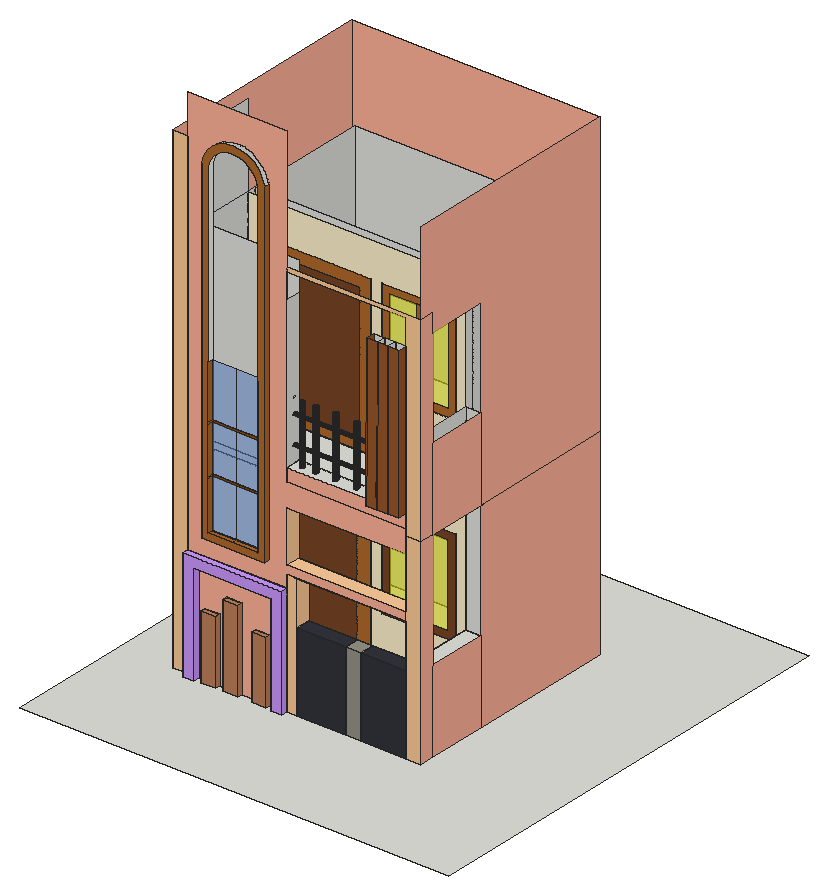
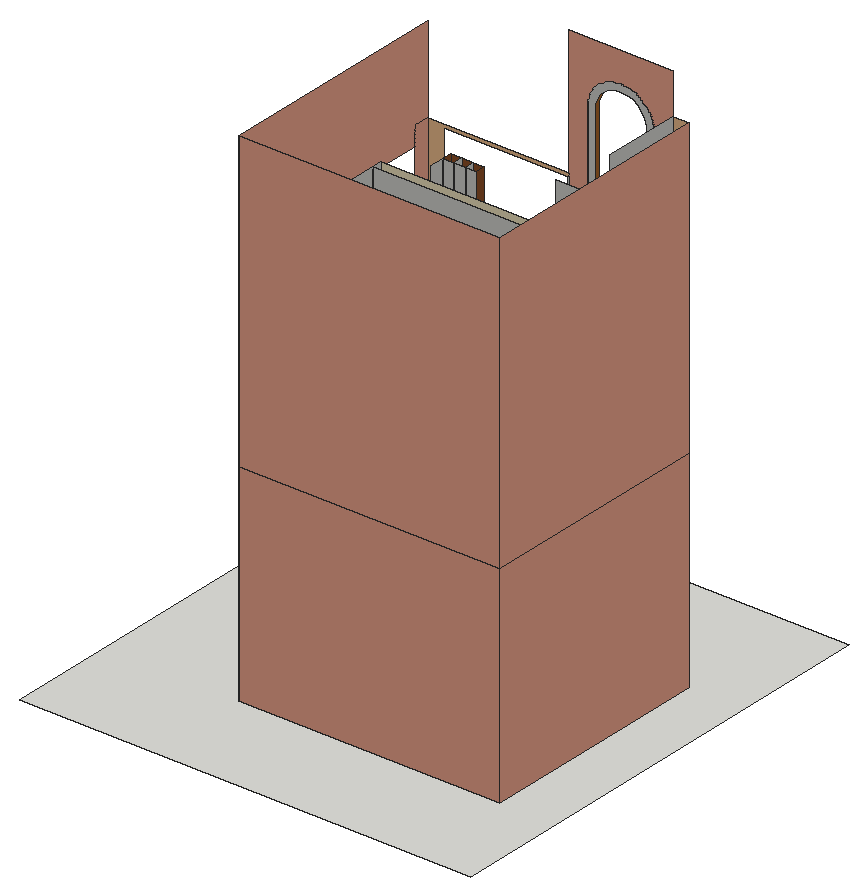
# SketchUp Ruby script. Lengths in inches.
U = 1.inch
M = Sketchup.active_model
def pt(a) = Geom::Point3d.new(a.map { |v| v * U })
def face(e, loops, mat)
  f = e.add_face(loops[0].map { |a| pt(a) })
  loops[1..].each { |l| e.add_face(l.map { |a| pt(a) }).erase! }
  f.material = f.back_material = mat if mat
  f
end
# faces: each face lists its corners as indices into pts; further lists are holes
def faces(e, pts, list, mat = nil) = list.each { |f| face(e, (f[0].is_a?(Array) ? f : [f]).map { |l| l.map { |i| pts[i] } }, mat) }
# xy, xz, yz: faces in a plane at the given z, y or x. An outline is a flat list of corners, or four numbers for a rectangle; further outlines are holes
def ring(l) = l.size == 4 ? [[l[0], l[1]], [l[2], l[1]], [l[2], l[3]], [l[0], l[3]]] : l.each_slice(2).to_a
def flat(e, list, mat, &to3) = list.each { |f| face(e, (f[0].is_a?(Array) ? f : [f]).map { |l| ring(l).map { |u, v| to3.(u, v) } }, mat) }
def xy(e, z, list, mat = nil) = flat(e, list, mat) { |x, y| [x, y, z] }
def xz(e, y, list, mat = nil) = flat(e, list, mat) { |x, z| [x, y, z] }
def yz(e, x, list, mat = nil) = flat(e, list, mat) { |y, z| [x, y, z] }
def lines(e, pts, list) = list.each { |a, b| e.add_line(pt(pts[a]), pt(pts[b])) }
# prism: a flat outline (further loops are holes) pulled along v
def prism(e, loops, v, mat = nil)
  f = face(e, loops, mat); d = Geom::Vector3d.new(v.map { |x| x * U })
  f.pushpull(f.normal.samedirection?(d) ? d.length : -d.length)
end
def box(e, o, s, mat = nil) = prism(e, [[o, [o[0] + s[0], o[1], o[2]], [o[0] + s[0], o[1] + s[1], o[2]], [o[0], o[1] + s[1], o[2]]]], [0, 0, s[2]], mat)
def at(x, y, z, deg = 0) = Geom::Transformation.translation(pt([x, y, z])) * Geom::Transformation.rotation(ORIGIN, Z_AXIS, deg.degrees)
def axes(o, x, y, z) = Geom::Transformation.new([*x, 0, *y, 0, *z, 0, *pt(o).to_a, 1])
def part(name) = M.definitions.add(name)
# library, detail: a bought-in or finely detailed component or shape, given as its bounding box
def library(name, o, s) = part(name).tap { |d| box(d.entities, o, s) }
def detail(e, o, s) = box(e.add_group.entities, o, s)
def put(e, d, t, mat = nil) = e.add_instance(d, t).tap { |i| i.material = mat if mat }
def group(e, t, mat = nil) = e.add_group.tap { |g| g.transformation = t; g.material = mat if mat }.entities
root = M.entities
M.materials.add("[Color B02]").color = [255, 178, 153]
M.materials.add("[Color C02]").color = [255, 204, 153]
M.materials.add("[Color C07]").color = [153, 76, 0]
M.materials.add("[Color D01]").color = [255, 242, 204]
M.materials.add("[Color J02]").color = [204, 153, 255]
M.materials.add("[Concrete Scored Jointless]").color = [140, 133, 127]
M.materials.add("[Formica Graystone]").color = [149, 146, 135]
M.materials.add("[Formica Laminate Dark]").color = [50, 53, 60]
M.materials.add("[Translucent Glass Blue]").color = [100, 149, 237]
M.materials["[Translucent Glass Blue]"].alpha = 0.5
M.materials.add("[Translucent Glass Gold]").color = [255, 254, 26]
M.materials["[Translucent Glass Gold]"].alpha = 0.6
M.materials.add("[Wood Bamboo]").color = [177, 105, 43]
M.materials.add("[Wood Cherry Original]").color = [152, 86, 42]
M.materials.add("[Wood Veneer 01]").color = [120, 70, 37]
M.materials.add("[Wood Veneer 02]").color = [190, 128, 91]
xy(root,0,[[[0,0,258.2,270.25],[31.82,74.84,40.82,74.84,40.82,83.84,100.51,83.84,100.51,74.84,181.07,74.84,181.07,210.03,31.82,210.03],[64.36,71.84,73.74,74.84],[81.64,71.84,90.64,74.84],[51.11,71.84,60.05,74.84],[40.82,70.96,47.66,74.84],[94.22,70.96,100.51,74.84]],[40.82,70.96,47.66,74.84],[94.22,70.96,100.51,74.84],[51.11,71.84,60.05,74.84],[64.36,71.84,73.74,74.84],
  [81.64,71.84,90.64,74.84],[31.82,74.84,40.82,119.85],[40.82,74.84,100.51,83.84],[100.51,74.84,106.7,83.84],[135.95,74.84,145.26,83.84],
  [172.07,74.84,181.07,83.84],[40.82,83.84,172.07,119.85],[172.07,83.84,181.07,119.85],[31.82,119.85,31.82,210.03,181.07,210.03,181.07,119.85,172.07,119.85,172.07,201.03,40.82,201.03,40.82,119.85],[40.82,119.85,62.57,125.32],
  [62.57,119.85,115.13,125.32],[115.13,119.85,172.07,125.32],[40.82,125.32,172.07,201.03]])
xy(root,0,[[106.7,74.84,135.95,83.84],[145.26,74.84,172.07,83.84]],"[Color C02]")
xy(root,38,[[81.64,71.84,90.64,74.84]],"[Wood Veneer 02]")
xy(root,38.625,[[51.11,71.84,60.05,74.84]],"[Wood Veneer 02]")
xy(root,40.68,[[122.02,119.85,166.34,125.32]])
xy(root,47.68,[[135.95,74.84,145.26,83.84]],"[Formica Graystone]")
xy(root,47.68,[[106.7,74.84,135.95,83.84],[145.26,74.84,172.07,83.84]],"[Formica Laminate Dark]")
xy(root,49.3125,[[64.36,71.84,73.74,74.84]],"[Wood Veneer 02]")
xy(root,49.8125,[[172.07,83.84,181.07,119.85]])
xy(root,60.76,[[47.66,70.96,94.22,74.84]])
xy(root,66.83,[[40.82,70.96,100.51,74.84]],"[Color J02]")
xy(root,74.33,[[100.51,74.84,106.7,83.84],[106.7,74.84,172.07,83.84]])
xy(root,78.07,[[51.65,71.71,89.65,74.84]])
xy(root,79.25,[[100.51,74.84,172.07,83.84]],"[Color C02]")
xy(root,82.18,[[55.76,71.71,70.65,74.84],[70.65,71.71,85.54,74.84]],"[Wood Bamboo]")
xy(root,99.0625,[[62.57,119.85,115.13,125.32]])
xy(root,99.5,[[122.02,119.85,166.34,125.32]])
xy(root,110.4375,[[100.51,74.84,111.08,83.84],[111.08,74.84,172.07,83.84]])
xy(root,120,[[172.07,74.84,181.07,83.84],[40.82,83.84,172.07,119.85],[172.07,83.84,181.07,119.85],[31.82,119.85,31.82,210.03,181.07,210.03,181.07,119.85,172.07,119.85,172.07,201.03,40.82,201.03,40.82,119.85],[40.82,119.85,62.57,125.32],
  [62.57,119.85,115.13,125.32],[115.13,119.85,172.07,125.32],[40.82,125.32,172.07,201.03]])
xy(root,123.9375,[[100.51,74.84,172.07,83.84],[40.82,83.84,172.07,119.85]])
xy(root,132,[[[100.51,74.84,172.07,83.84],[105.81,78.53,105.47,78.58,105.15,78.71,104.88,78.92,104.67,79.19,104.54,79.51,104.5,79.85,104.54,80.1875,104.67,80.5,104.88,80.77,105.15,80.98,105.47,81.11,105.81,81.16,106.15,81.11,106.46,80.98,106.74,80.77,106.95,80.5,107.08,80.1875,107.12,79.85,107.08,79.51,106.95,79.19,106.74,78.92,106.46,78.71,106.15,78.58],[151.93,78.53,151.59,78.58,151.28,78.71,151.01,78.92,150.8,79.19,150.67,79.51,150.62,79.85,150.67,80.1875,150.8,80.5,151.01,80.77,151.28,80.98,151.59,81.11,151.93,81.16,152.27,81.11,152.59,80.98,152.86,80.77,153.07,80.5,153.2,80.1875,153.25,79.85,153.2,79.51,153.07,79.19,152.86,78.92,152.59,78.71,152.27,78.58],[138.62,78.53,138.28,78.58,137.96,78.71,137.69,78.92,137.48,79.19,137.35,79.51,137.31,79.85,137.35,80.1875,137.48,80.5,137.69,80.77,137.96,80.98,138.28,81.11,138.62,81.16,138.96,81.11,139.28,80.98,139.55,80.77,139.76,80.5,139.89,80.1875,139.93,79.85,139.89,79.51,139.76,79.19,139.55,78.92,139.28,78.71,138.96,78.58],[126,78.53,125.66,78.58,125.34,78.71,125.07,78.92,124.86,79.19,124.73,79.51,124.68,79.85,124.73,80.1875,124.86,80.5,125.07,80.77,125.34,80.98,125.66,81.11,126,81.16,126.34,81.11,126.65,80.98,126.92,80.77,127.13,80.5,127.26,80.1875,127.31,79.85,127.26,79.51,127.13,79.19,126.92,78.92,126.65,78.71,126.34,78.58],[114.06,78.53,113.72,78.58,113.4,78.71,113.13,78.92,112.92,79.19,112.79,79.51,112.75,79.85,112.79,80.1875,112.92,80.5,113.13,80.77,113.4,80.98,113.72,81.11,114.06,81.16,114.4,81.11,114.71,80.98,114.99,80.77,115.2,80.5,115.33,80.1875,115.37,79.85,115.33,79.51,115.2,79.19,114.99,78.92,114.71,78.71,114.4,78.58]],[105.81,78.53,105.47,78.58,105.15,78.71,104.88,78.92,104.67,79.19,104.54,79.51,104.5,79.85,104.54,80.1875,104.67,80.5,104.88,80.77,105.15,80.98,105.47,81.11,105.81,81.16,106.15,81.11,106.46,80.98,106.74,80.77,106.95,80.5,107.08,80.1875,107.12,79.85,107.08,79.51,106.95,79.19,106.74,78.92,106.46,78.71,106.15,78.58],[114.06,78.53,113.72,78.58,113.4,78.71,113.13,78.92,112.92,79.19,112.79,79.51,112.75,79.85,112.79,80.1875,112.92,80.5,113.13,80.77,113.4,80.98,113.72,81.11,114.06,81.16,114.4,81.11,114.71,80.98,114.99,80.77,115.2,80.5,115.33,80.1875,115.37,79.85,115.33,79.51,115.2,79.19,114.99,78.92,114.71,78.71,114.4,78.58],[126,78.53,125.66,78.58,125.34,78.71,125.07,78.92,124.86,79.19,124.73,79.51,124.68,79.85,124.73,80.1875,124.86,80.5,125.07,80.77,125.34,80.98,125.66,81.11,126,81.16,126.34,81.11,126.65,80.98,126.92,80.77,127.13,80.5,127.26,80.1875,127.31,79.85,127.26,79.51,127.13,79.19,126.92,78.92,126.65,78.71,126.34,78.58],[138.62,78.53,138.28,78.58,137.96,78.71,137.69,78.92,137.48,79.19,137.35,79.51,137.31,79.85,137.35,80.1875,137.48,80.5,137.69,80.77,137.96,80.98,138.28,81.11,138.62,81.16,138.96,81.11,139.28,80.98,139.55,80.77,139.76,80.5,139.89,80.1875,139.93,79.85,139.89,79.51,139.76,79.19,139.55,78.92,139.28,78.71,138.96,78.58],
  [151.93,78.53,151.59,78.58,151.28,78.71,151.01,78.92,150.8,79.19,150.67,79.51,150.62,79.85,150.67,80.1875,150.8,80.5,151.01,80.77,151.28,80.98,151.59,81.11,151.93,81.16,152.27,81.11,152.59,80.98,152.86,80.77,153.07,80.5,153.2,80.1875,153.25,79.85,153.2,79.51,153.07,79.19,152.86,78.92,152.59,78.71,152.27,78.58]])
xy(root,160.68,[[122.02,119.85,166.34,125.32]])
xz(root,70.96,[[40.82,0,47.66,0,47.66,60.76,94.22,60.76,94.22,0,100.51,0,100.51,66.83,40.82,66.83]],"[Color J02]")
xz(root,71.71,[[[51.65,78.07,89.65,78.07,89.65,280.57,88.3,284.79,86.03,288.59,82.95,291.78,79.23,294.18,75.05,295.68,70.65,296.18,66.25,295.68,62.08,294.18,58.35,291.78,55.28,288.59,53,284.79,51.65,280.57],[55.76,82.18,55.76,279.92,56.77,283.08,58.5625,286.07,60.98,288.58,63.91,290.47,67.19,291.64,70.65,292.04,74.11,291.64,77.39,290.47,80.32,288.58,82.74,286.07,84.53,283.08,85.54,279.92,85.54,82.18]]],"[Wood Bamboo]")
xz(root,71.84,[[51.11,0,60.05,38.625],[64.36,0,73.74,49.3125],[81.64,0,90.64,38]],"[Wood Veneer 02]")
xz(root,74.84,[[40.82,0,40.82,66.83,100.51,66.83,100.51,0,94.22,0,94.22,60.76,47.66,60.76,47.66,0],[51.11,0,60.05,38.625],[64.36,0,73.74,49.3125],[81.64,0,90.64,38],[[51.65,78.07,51.65,280.57,53,284.79,55.28,288.59,58.35,291.78,62.08,294.18,66.25,295.68,70.65,296.18,75.05,295.68,79.23,294.18,82.95,291.78,86.03,288.59,88.3,284.79,89.65,280.57,89.65,78.07],[55.76,82.18,85.54,82.18,85.54,279.92,84.53,283.08,82.74,286.07,80.32,288.58,77.39,290.47,74.11,291.64,70.65,292.04,67.19,291.64,63.91,290.47,60.98,288.58,58.5625,286.07,56.77,283.08,55.76,279.92]]])
xz(root,74.84,[[47.66,0,51.11,0,51.11,38.625,60.05,38.625,60.05,0,64.36,0,64.36,49.3125,73.74,49.3125,73.74,0,81.64,0,81.64,38,90.64,38,90.64,0,94.22,0,94.22,60.76,47.66,60.76],[[40.82,66.83,100.51,66.83,100.51,74.33,172.07,74.33,172.07,79.25,100.51,79.25,100.51,110.4375,172.07,110.4375,172.07,123.9375,100.51,123.9375,100.51,313.4,40.82,313.4],[51.65,78.07,51.65,280.57,53,284.79,55.28,288.59,58.35,291.78,62.08,294.18,66.25,295.68,70.65,296.18,75.05,295.68,79.23,294.18,82.95,291.78,86.03,288.59,88.3,284.79,89.65,280.57,89.65,78.07]],[100.51,123.9375,172.07,132]],"[Color B02]")
xz(root,74.84,[[31.82,0,40.82,289.8125],[100.51,0,106.7,74.33],[172.07,0,181.07,120],[172.07,120,181.07,120,181.07,240,100.51,240,100.51,237.59,172.07,237.59]],"[Color C02]")
xz(root,74.84,[[55.76,111.46,70.65,112.71],[70.65,111.46,85.54,112.71],[55.76,140.74,70.65,142],[70.65,140.74,85.54,142]],"[Color C07]")
xz(root,74.84,[[135.95,0,145.26,47.68]],"[Formica Graystone]")
xz(root,74.84,[[106.7,0,135.95,47.68],[145.26,0,172.07,47.68]],"[Formica Laminate Dark]")
xz(root,74.84,[[55.76,82.18,70.65,111.46],[70.65,82.18,85.54,111.46],[55.76,112.71,70.65,140.74],[70.65,112.71,85.54,140.74],[55.76,142,70.65,174.43],
  [70.65,142,85.54,174.43]],"[Translucent Glass Blue]")
xz(root,83.84,[[40.82,0,40.82,120,100.51,120,100.51,79.25,172.07,79.25,172.07,74.33,100.51,74.33,100.51,0],[100.51,0,106.7,74.33],[135.95,0,145.26,47.68],[172.07,0,181.07,49.8125],[172.07,49.8125,181.07,120],
  [100.51,110.4375,111.08,120],[111.08,110.4375,172.07,120],[40.82,120,111.08,123.9375],[111.08,120,172.07,123.9375],[172.07,120,181.07,169.8125],
  [40.82,123.9375,100.51,240],[100.51,123.9375,111.08,132],[111.08,123.9375,172.07,132]])
xz(root,83.84,[[106.7,0,135.95,47.68],[145.26,0,172.07,47.68]],"[Color C02]")
xz(root,119.85,[[172.07,0,181.07,49.8125],[172.07,49.8125,181.07,120],[40.82,120,62.57,123.9375],[62.57,120,115.13,123.9375],[115.13,120,172.07,123.9375],
  [172.07,120,181.07,169.8125]])
xz(root,119.85,[[[40.82,0,62.57,0,62.57,99.0625,115.13,99.0625,115.13,0,172.07,0,172.07,120,40.82,120],[122.02,40.68,166.34,99.5]],[[40.82,123.9375,62.57,123.9375,62.57,219.0625,115.13,219.0625,115.13,123.9375,172.07,123.9375,172.07,240,40.82,240],[122.02,160.68,166.34,219.5]]],"[Color D01]")
xz(root,119.85,[[126.67,45.33,141.29,94.85],[145.9,45.33,161.69,94.85],[126.53,165.1875,142.55,214.99],[146.36,165.1875,161.83,214.99]],"[Translucent Glass Gold]")
xz(root,119.85,[[[62.57,0,115.13,99.0625],[71.2,8.63,106.5,90.43]],[[62.57,123.9375,115.13,219.0625],[69.44,130.8125,108.26,212.1875]],[[122.02,160.68,166.34,219.5],[126.53,165.1875,161.83,214.99]],[142.55,165.1875,146.36,214.99]],"[Wood Bamboo]")
xz(root,119.85,[[71.2,8.63,106.5,90.43],[[122.02,40.68,166.34,99.5],[126.67,45.33,161.69,94.85]],[141.29,45.33,145.9,94.85],[69.44,130.8125,108.26,212.1875]],"[Wood Veneer 01]")
xz(root,125.32,[[[40.82,0,40.82,120,172.07,120,172.07,0,115.13,0,115.13,99.0625,62.57,99.0625,62.57,0],[122.02,40.68,166.34,99.5]],[[40.82,120,40.82,240,172.07,240,172.07,120,115.13,120,115.13,219.0625,62.57,219.0625,62.57,120],[122.02,160.68,166.34,219.5]]])
xz(root,201.03,[[40.82,0,172.07,120],[40.82,120,172.07,240]])
xz(root,210.03,[[31.82,0,181.07,120],[31.82,120,181.07,289.8125]],"[Color B02]")
yz(root,31.82,[[74.84,0,210.03,120],[74.84,120,210.03,289.8125]],"[Color B02]")
yz(root,40.82,[[74.84,0,83.84,120],[83.84,0,119.85,120],[119.85,0,125.32,120],[125.32,0,201.03,120],[74.84,120,83.84,123.9375],
  [83.84,120,119.85,123.9375],[119.85,120,125.32,240],[125.32,120,201.03,240],[74.84,123.9375,83.84,123.9375,83.84,240,119.85,240,119.85,289.8125,74.84,289.8125],[83.84,123.9375,119.85,240]])
yz(root,40.82,[[70.96,0,74.84,66.83]],"[Color J02]")
yz(root,47.66,[[70.96,0,74.84,60.76]],"[Color J02]")
yz(root,51.11,[[71.84,0,74.84,38.625]],"[Wood Veneer 02]")
yz(root,51.65,[[71.71,78.07,74.84,280.57]],"[Wood Bamboo]")
yz(root,55.76,[[71.71,82.18,74.84,111.46],[71.71,111.46,74.84,112.71],[71.71,112.71,74.84,140.74],[71.71,140.74,74.84,142],[71.71,142,74.84,174.43]],"[Wood Bamboo]")
yz(root,60.05,[[71.84,0,74.84,38.625]],"[Wood Veneer 02]")
yz(root,62.57,[[119.85,0,125.32,99.0625],[119.85,120,125.32,219.0625]])
yz(root,64.36,[[71.84,0,74.84,49.3125]],"[Wood Veneer 02]")
yz(root,73.74,[[71.84,0,74.84,49.3125]],"[Wood Veneer 02]")
yz(root,81.64,[[71.84,0,74.84,38]],"[Wood Veneer 02]")
yz(root,85.54,[[71.71,82.18,74.84,111.46],[71.71,111.46,74.84,112.71],[71.71,112.71,74.84,140.74],[71.71,140.74,74.84,142],[71.71,142,74.84,174.43]],"[Wood Bamboo]")
yz(root,89.65,[[71.71,78.07,74.84,280.57]],"[Wood Bamboo]")
yz(root,90.64,[[71.84,0,74.84,38]],"[Wood Veneer 02]")
yz(root,94.22,[[70.96,0,74.84,60.76]],"[Color J02]")
yz(root,100.51,[[74.84,0,83.84,74.33],[74.84,123.9375,83.84,132],[[74.84,132,83.84,132,83.84,222.27,75.28,222.27,75.28,237.59,74.84,237.59],[80.44,166.375,80.17,166.41,79.91,166.52,79.69,166.68,79.52,166.9,79.42,167.16,79.38,167.4375,79.42,167.71,79.52,167.97,79.69,168.1875,79.91,168.36,80.17,168.46,80.44,168.5,80.72,168.46,80.97,168.36,81.19,168.1875,81.36,167.97,81.47,167.71,81.51,167.4375,81.47,167.16,81.36,166.9,81.19,166.68,80.97,166.52,80.72,166.41],[80.22,157.93,80,157.96,79.78,158.05,79.6,158.1875,79.46,158.37,79.38,158.58,79.35,158.81,79.38,159.03,79.46,159.24,79.6,159.43,79.78,159.57,80,159.65,80.22,159.68,80.45,159.65,80.66,159.57,80.84,159.43,80.98,159.24,81.07,159.03,81.1,158.81,81.07,158.58,80.98,158.37,80.84,158.1875,80.66,158.05,80.45,157.96],[80.22,141.24,80,141.27,79.78,141.36,79.6,141.5,79.46,141.68,79.38,141.89,79.35,142.12,79.38,142.35,79.46,142.56,79.6,142.74,79.78,142.88,80,142.97,80.22,142.99,80.45,142.97,80.66,142.88,80.84,142.74,80.98,142.56,81.07,142.35,81.1,142.12,81.07,141.89,80.98,141.68,80.84,141.5,80.66,141.36,80.45,141.27]],[80.22,141.24,80,141.27,79.78,141.36,79.6,141.5,79.46,141.68,79.38,141.89,79.35,142.12,79.38,142.35,79.46,142.56,79.6,142.74,79.78,142.88,80,142.97,80.22,142.99,80.45,142.97,80.66,142.88,80.84,142.74,80.98,142.56,81.07,142.35,81.1,142.12,81.07,141.89,80.98,141.68,80.84,141.5,80.66,141.36,80.45,141.27],[80.22,157.93,80,157.96,79.78,158.05,79.6,158.1875,79.46,158.37,79.38,158.58,79.35,158.81,79.38,159.03,79.46,159.24,79.6,159.43,79.78,159.57,80,159.65,80.22,159.68,80.45,159.65,80.66,159.57,80.84,159.43,80.98,159.24,81.07,159.03,81.1,158.81,81.07,158.58,80.98,158.37,80.84,158.1875,80.66,158.05,80.45,157.96]])
yz(root,100.51,[[74.84,79.25,83.84,110.4375]],"[Color C02]")
yz(root,100.51,[[70.96,0,74.84,66.83]],"[Color J02]")
yz(root,106.7,[[74.84,0,83.84,47.68],[74.84,47.68,83.84,74.33]],"[Color C02]")
yz(root,115.13,[[119.85,0,125.32,99.0625],[119.85,120,125.32,219.0625]])
yz(root,122.02,[[119.85,40.68,125.32,99.5],[119.85,160.68,125.32,219.5]])
yz(root,135.95,[[74.84,0,83.84,47.68]],"[Color C02]")
yz(root,145.26,[[74.84,0,83.84,47.68]],"[Color C02]")
yz(root,152.68,[[74.84,132,69.46,132.03,69.9,222.3,75.28,222.27]],"[Wood Cherry Original]")
yz(root,159.14,[[74.84,132,75.28,222.27,69.9,222.3,69.46,132.03]])
yz(root,165.61,[[74.84,132,75.28,222.27,69.9,222.3,69.46,132.03]])
yz(root,166.34,[[119.85,40.68,125.32,99.5],[119.85,160.68,125.32,219.5]])
yz(root,172.07,[[83.84,0,119.85,49.8125],[119.85,0,125.32,120],[125.32,0,201.03,120],[74.84,110.4375,83.84,120],[74.84,120,83.84,123.9375],
  [83.84,120,119.85,123.9375],[119.85,120,125.32,240],[125.32,120,201.03,240],[74.84,123.9375,83.84,132],[83.84,123.9375,119.85,169.8125],
  [74.84,132,75.28,222.27,74.84,222.27],[74.84,132,75.28,222.27,75.28,132],[75.28,132,83.84,222.27]])
yz(root,172.07,[[74.84,0,83.84,47.68],[74.84,47.68,83.84,74.33],[74.84,79.25,83.84,110.4375]],"[Color C02]")
yz(root,172.07,[[74.84,132,74.84,222.28,69.9,222.3,69.46,132.03]],"[Wood Cherry Original]")
yz(root,172.2,[[80.22,141.24,80.45,141.27,80.66,141.36,80.84,141.5,80.98,141.68,81.07,141.89,81.1,142.12,81.07,142.35,80.98,142.56,80.84,142.74,80.66,142.88,80.45,142.97,80.22,142.99,80,142.97,79.78,142.88,79.6,142.74,79.46,142.56,79.38,142.35,79.35,142.12,79.38,141.89,79.46,141.68,79.6,141.5,79.78,141.36,80,141.27],[80.22,157.93,80.45,157.96,80.66,158.05,80.84,158.1875,80.98,158.37,81.07,158.58,81.1,158.81,81.07,159.03,80.98,159.24,80.84,159.43,80.66,159.57,80.45,159.65,80.22,159.68,80,159.65,79.78,159.57,79.6,159.43,79.46,159.24,79.38,159.03,79.35,158.81,79.38,158.58,79.46,158.37,79.6,158.1875,79.78,158.05,80,157.96]])
yz(root,181.07,[[74.84,0,83.84,120],[83.84,0,119.85,49.8125],[119.85,0,210.03,120],[119.85,120,210.03,120,210.03,289.8125,74.84,289.8125,74.84,240,83.84,240,83.84,229.05,119.85,229.05],[74.84,120,83.84,240],
  [83.84,120,119.85,169.8125]],"[Color B02]")
p = [[152.68,74.84,132],[159.14,74.84,132],[159.14,69.46,132.03],[152.68,69.46,132.03],[159.14,69.9,222.3],[152.68,69.9,222.3],
  [165.61,74.84,132],[165.61,69.46,132.03],[165.61,69.9,222.3],[172.07,74.84,132],[172.07,69.46,132.03],[172.07,69.9,222.3],
  [159.14,75.28,222.27],[152.68,75.28,222.27],[165.61,75.28,222.27],[172.07,75.28,222.27],[105.47,78.58,132],[105.81,78.53,132],
  [105.81,78.53,167.16],[105.47,78.58,167.16],[106.15,78.58,132],[106.15,78.58,167.16],[113.72,78.58,132],[114.06,78.53,132],
  [114.06,78.53,167.4375],[113.72,78.58,167.4375],[114.4,78.58,132],[114.4,78.58,167.4375],[125.66,78.58,132],[126,78.53,132],
  [126,78.53,167.97],[125.66,78.58,167.97],[126.34,78.58,132],[126.34,78.58,167.97],[138.28,78.58,132],[138.62,78.53,132],
  [138.62,78.53,167.4375],[138.28,78.58,167.4375],[138.96,78.58,132],[138.96,78.58,167.4375],[151.59,78.58,132],[151.93,78.53,132],
  [151.93,78.53,167.4375],[151.59,78.58,167.4375],[152.27,78.58,132],[152.27,78.58,167.4375],[105.15,78.71,132],[105.15,78.71,167.16],
  [106.46,78.71,132],[106.46,78.71,167.16],[113.4,78.71,132],[113.4,78.71,167.4375],[114.71,78.71,132],[114.71,78.71,167.4375],
  [125.34,78.71,132],[125.34,78.71,167.97],[126.65,78.71,132],[126.65,78.71,167.97],[137.96,78.71,132],[137.96,78.71,167.4375],
  [139.28,78.71,132],[139.28,78.71,167.4375],[151.28,78.71,132],[151.28,78.71,167.4375],[152.59,78.71,132],[152.59,78.71,167.4375],
  [104.88,78.92,132],[104.88,78.92,167.16],[106.74,78.92,132],[106.74,78.92,167.16],[113.13,78.92,132],[113.13,78.92,167.4375],
  [114.99,78.92,132],[114.99,78.92,167.4375],[125.07,78.92,132],[125.07,78.92,167.97],[126.92,78.92,132],[126.92,78.92,167.97],
  [137.69,78.92,132],[137.69,78.92,167.4375],[139.55,78.92,132],[139.55,78.92,167.4375],[151.01,78.92,132],[151.01,78.92,167.4375],
  [152.86,78.92,132],[152.86,78.92,167.4375],[104.67,79.19,132],[104.67,79.19,167.16],[106.95,79.19,132],[106.95,79.19,167.16],
  [112.92,79.19,132],[112.92,79.19,167.4375],[115.2,79.19,132],[115.2,79.19,167.4375],[124.86,79.19,132],[124.86,79.19,167.97],
  [127.13,79.19,132],[127.13,79.19,167.97],[137.48,79.19,132],[137.48,79.19,167.4375],[139.76,79.19,132],[139.76,79.19,167.4375],
  [150.8,79.19,132],[150.8,79.19,167.4375],[153.07,79.19,132],[153.07,79.19,167.4375],[104.54,79.51,132],[104.58,79.42,167.16],
  [104.54,79.51,167.16],[107.08,79.51,132],[107.08,79.51,167.16],[107.04,79.42,167.16],[112.79,79.51,132],[112.84,79.38,167.4375],
  [112.79,79.51,167.4375],[115.33,79.51,132],[115.33,79.51,167.4375],[115.27,79.38,167.4375],[124.73,79.51,132],[124.73,79.51,167.97],
  [127.26,79.51,132],[127.26,79.51,167.97],[137.35,79.51,132],[137.41,79.38,167.4375],[137.35,79.51,167.4375],[139.89,79.51,132],
  [139.89,79.51,167.4375],[139.84,79.38,167.4375],[150.67,79.51,132],[150.72,79.38,167.4375],[150.67,79.51,167.4375],[153.2,79.51,132],
  [153.2,79.51,167.4375],[153.15,79.38,167.4375],[104.5,79.85,132],[104.5,79.85,167.16],[107.12,79.85,132],[107.12,79.85,167.16],
  [112.75,79.85,132],[112.75,79.85,167.4375],[115.37,79.85,132],[115.37,79.85,167.4375],[124.68,79.85,132],[124.73,79.52,167.97],
  [124.68,79.85,167.97],[127.31,79.85,132],[127.31,79.85,167.97],[127.27,79.52,167.97],[137.31,79.85,132],[137.31,79.85,167.4375],
  [139.93,79.85,132],[139.93,79.85,167.4375],[150.62,79.85,132],[150.62,79.85,167.4375],[153.25,79.85,132],[153.25,79.85,167.4375],
  [104.54,80.1875,132],[104.54,80.1875,167.16],[107.08,80.1875,132],[107.08,80.1875,167.16],[112.79,80.1875,132],[112.79,80.1875,167.4375],
  [115.33,80.1875,132],[115.33,80.1875,167.4375],[124.73,80.1875,132],[124.73,80.1875,167.97],[127.26,80.1875,132],[127.26,80.1875,167.97],
  [137.35,80.1875,132],[137.35,80.1875,167.4375],[139.89,80.1875,132],[139.89,80.1875,167.4375],[150.67,80.1875,132],[150.67,80.1875,167.4375],
  [153.2,80.1875,132],[153.2,80.1875,167.4375],[104.67,80.5,132],[104.67,80.5,167.16],[106.95,80.5,132],[106.95,80.5,167.16],
  [112.92,80.5,132],[112.92,80.5,167.4375],[115.2,80.5,132],[115.2,80.5,167.4375],[124.86,80.5,132],[124.86,80.5,167.97],
  [127.13,80.5,132],[127.13,80.5,167.97],[137.48,80.5,132],[137.48,80.5,167.4375],[139.76,80.5,132],[139.76,80.5,167.4375],
  [150.8,80.5,132],[150.8,80.5,167.4375],[153.07,80.5,132],[153.07,80.5,167.4375],[104.88,80.77,132],[104.88,80.77,167.16],
  [106.74,80.77,132],[106.74,80.77,167.16],[113.13,80.77,132],[113.13,80.77,167.4375],[114.99,80.77,132],[114.99,80.77,167.4375],
  [125.07,80.77,132],[125.07,80.77,167.97],[126.92,80.77,132],[126.92,80.77,167.97],[137.69,80.77,132],[137.69,80.77,167.4375],
  [139.55,80.77,132],[139.55,80.77,167.4375],[151.01,80.77,132],[151.01,80.77,167.4375],[152.86,80.77,132],[152.86,80.77,167.4375],
  [105.15,80.98,132],[105.15,80.98,167.16],[106.46,80.98,132],[106.46,80.98,167.16],[113.4,80.98,132],[113.4,80.98,167.4375],
  [114.71,80.98,132],[114.71,80.98,167.4375],[125.34,80.98,132],[125.34,80.98,167.97],[126.65,80.98,132],[126.65,80.98,167.97],
  [137.96,80.98,132],[137.96,80.98,167.4375],[139.28,80.98,132],[139.28,80.98,167.4375],[151.28,80.98,132],[151.28,80.98,167.4375],
  [152.59,80.98,132],[152.59,80.98,167.4375],[105.47,81.11,132],[105.47,81.11,167.16],[106.15,81.11,132],[106.15,81.11,167.16],
  [113.72,81.11,132],[113.72,81.11,167.4375],[114.4,81.11,132],[114.4,81.11,167.4375],[125.66,81.11,132],[125.66,81.11,167.97],
  [126.34,81.11,132],[126.34,81.11,167.97],[138.28,81.11,132],[138.28,81.11,167.4375],[138.96,81.11,132],[138.96,81.11,167.4375],
  [151.59,81.11,132],[151.59,81.11,167.4375],[152.27,81.11,132],[152.27,81.11,167.4375],[105.81,81.16,132],[105.81,81.16,167.16],
  [114.06,81.16,132],[114.06,81.16,167.4375],[126,81.16,132],[126,81.16,167.97],[138.62,81.16,132],[138.62,81.16,167.4375],
  [151.93,81.16,132],[151.93,81.16,167.4375],[100.51,80,141.27],[100.51,80.22,141.24],[172.2,80.22,141.24],[172.2,80,141.27],
  [100.51,80.45,141.27],[172.2,80.45,141.27],[100.51,79.78,141.36],[172.2,79.78,141.36],[100.51,80.66,141.36],[172.2,80.66,141.36],
  [100.51,79.6,141.5],[172.2,79.6,141.5],[100.51,80.84,141.5],[172.2,80.84,141.5],[100.51,79.46,141.68],[172.2,79.46,141.68],
  [100.51,80.98,141.68],[172.2,80.98,141.68],[100.51,79.38,141.89],[172.2,79.38,141.89],[100.51,81.07,141.89],[172.2,81.07,141.89],
  [100.51,79.35,142.12],[172.2,79.35,142.12],[100.51,81.1,142.12],[172.2,81.1,142.12],[100.51,79.38,142.35],[172.2,79.38,142.35],
  [100.51,81.07,142.35],[172.2,81.07,142.35],[100.51,79.46,142.56],[172.2,79.46,142.56],[100.51,80.98,142.56],[172.2,80.98,142.56],
  [100.51,79.6,142.74],[172.2,79.6,142.74],[100.51,80.84,142.74],[172.2,80.84,142.74],[100.51,79.78,142.88],[172.2,79.78,142.88],
  [100.51,80.66,142.88],[172.2,80.66,142.88],[100.51,80,142.97],[172.2,80,142.97],[100.51,80.45,142.97],[172.2,80.45,142.97],
  [100.51,80.22,142.99],[172.2,80.22,142.99],[100.51,80,157.96],[100.51,80.22,157.93],[172.2,80.22,157.93],[172.2,80,157.96],
  [100.51,80.45,157.96],[172.2,80.45,157.96],[100.51,79.6,158.1875],[100.51,79.78,158.05],[172.2,79.78,158.05],[172.2,79.6,158.1875],
  [100.51,80.66,158.05],[172.2,80.66,158.05],[100.51,80.84,158.1875],[172.2,80.84,158.1875],[100.51,79.46,158.37],[172.2,79.46,158.37],
  [100.51,80.98,158.37],[172.2,80.98,158.37],[100.51,79.38,158.58],[172.2,79.38,158.58],[100.51,81.07,158.58],[172.2,81.07,158.58],
  [100.51,79.35,158.81],[172.2,79.35,158.81],[100.51,81.1,158.81],[172.2,81.1,158.81],[100.51,79.38,159.03],[172.2,79.38,159.03],
  [100.51,81.07,159.03],[172.2,81.07,159.03],[100.51,79.46,159.24],[172.2,79.46,159.24],[100.51,80.98,159.24],[172.2,80.98,159.24],
  [100.51,79.6,159.43],[172.2,79.6,159.43],[100.51,80.84,159.43],[172.2,80.84,159.43],[100.51,79.78,159.57],[172.2,79.78,159.57],
  [100.51,80.66,159.57],[172.2,80.66,159.57],[100.51,80,159.65],[172.2,80,159.65],[100.51,80.45,159.65],[172.2,80.45,159.65],
  [100.51,80.22,159.68],[172.2,80.22,159.68],[165.61,74.84,222.27],[159.14,74.84,222.27]]
faces(root,p,[[0,1,2,3],[2,4,5,3],[1,6,7,2],[7,8,4,2],[6,9,10,7],[10,11,8,7]],"[Wood Cherry Original]")
faces(root,p,[[12,1,0,13],[14,6,1,12],[15,9,6,14]])
faces(root,p,[[16,17,18,19],[17,20,21,18],[22,23,24,25],[23,26,27,24],[28,29,30,31],[29,32,33,30],[34,35,36,37],[35,38,39,36],
  [40,41,42,43],[41,44,45,42],[46,16,19,47],[20,48,49,21],[50,22,25,51],[26,52,53,27],[54,28,31,55],[32,56,57,33],
  [58,34,37,59],[38,60,61,39],[62,40,43,63],[44,64,65,45],[66,46,47,67],[48,68,69,49],[70,50,51,71],[52,72,73,53],
  [74,54,55,75],[56,76,77,57],[78,58,59,79],[60,80,81,61],[82,62,63,83],[64,84,85,65],[86,66,67,87],[68,88,89,69],
  [90,70,71,91],[72,92,93,73],[94,74,75,95],[76,96,97,77],[98,78,79,99],[80,100,101,81],[102,82,83,103],[84,104,105,85],
  [106,86,87,107,108],[88,109,110,111,89],[112,90,91,113,114],[92,115,116,117,93],[118,94,95,119],[96,120,121,97],[122,98,99,123,124],[100,125,126,127,101],
  [128,102,103,129,130],[104,131,132,133,105],[134,106,108,135],[109,136,137,110],[138,112,114,139],[115,140,141,116],[142,118,119,143,144],[120,145,146,147,121],
  [148,122,124,149],[125,150,151,126],[152,128,130,153],[131,154,155,132],[156,134,135,157],[136,158,159,137],[160,138,139,161],[140,162,163,141],
  [164,142,144,165],[145,166,167,146],[168,148,149,169],[150,170,171,151],[172,152,153,173],[154,174,175,155],[176,156,157,177],[158,178,179,159],
  [180,160,161,181],[162,182,183,163],[184,164,165,185],[166,186,187,167],[188,168,169,189],[170,190,191,171],[192,172,173,193],[174,194,195,175],
  [196,176,177,197],[178,198,199,179],[200,180,181,201],[182,202,203,183],[204,184,185,205],[186,206,207,187],[208,188,189,209],[190,210,211,191],
  [212,192,193,213],[194,214,215,195],[216,196,197,217],[198,218,219,199],[220,200,201,221],[202,222,223,203],[224,204,205,225],[206,226,227,207],
  [228,208,209,229],[210,230,231,211],[232,212,213,233],[214,234,235,215],[236,216,217,237],[218,238,239,219],[240,220,221,241],[222,242,243,223],
  [244,224,225,245],[226,246,247,227],[248,228,229,249],[230,250,251,231],[252,232,233,253],[234,254,255,235],[256,236,237,257],[238,256,257,239],
  [258,240,241,259],[242,258,259,243],[260,244,245,261],[246,260,261,247],[262,248,249,263],[250,262,263,251],[264,252,253,265],[254,264,265,255],
  [266,267,268,269],[267,270,271,268],[272,266,269,273],[270,274,275,271],[276,272,273,277],[274,278,279,275],[280,276,277,281],[278,282,283,279],
  [284,280,281,285],[282,286,287,283],[288,284,285,289],[286,290,291,287],[292,288,289,293],[290,294,295,291],[296,292,293,297],[294,298,299,295],
  [300,296,297,301],[298,302,303,299],[304,300,301,305],[302,306,307,303],[308,304,305,309],[306,310,311,307],[312,308,309,313],[310,312,313,311],
  [314,315,316,317],[315,318,319,316],[320,321,322,323],[321,314,317,322],[318,324,325,319],[324,326,327,325],[328,320,323,329],[326,330,331,327],
  [332,328,329,333],[330,334,335,331],[336,332,333,337],[334,338,339,335],[340,336,337,341],[338,342,343,339],[344,340,341,345],[342,346,347,343],
  [348,344,345,349],[346,350,351,347],[352,348,349,353],[350,354,355,351],[356,352,353,357],[354,358,359,355],[360,356,357,361],[358,360,361,359]],"[Concrete Scored Jointless]")
lines(root,p,[[6,362],[1,363]])
